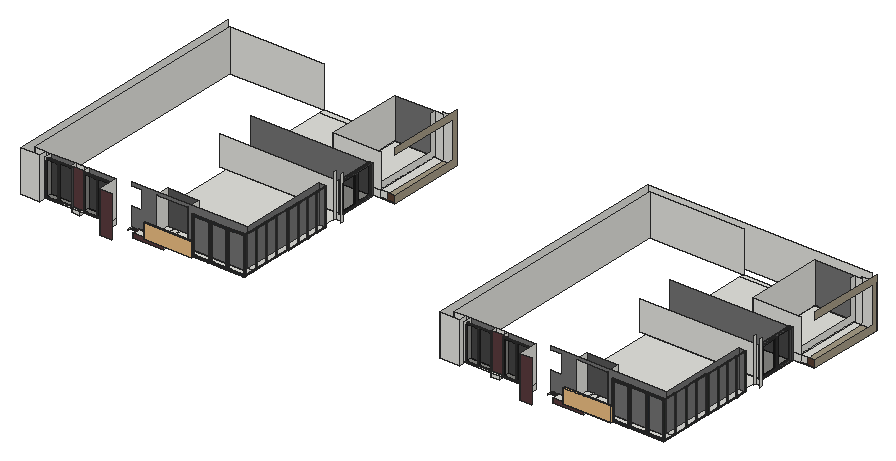
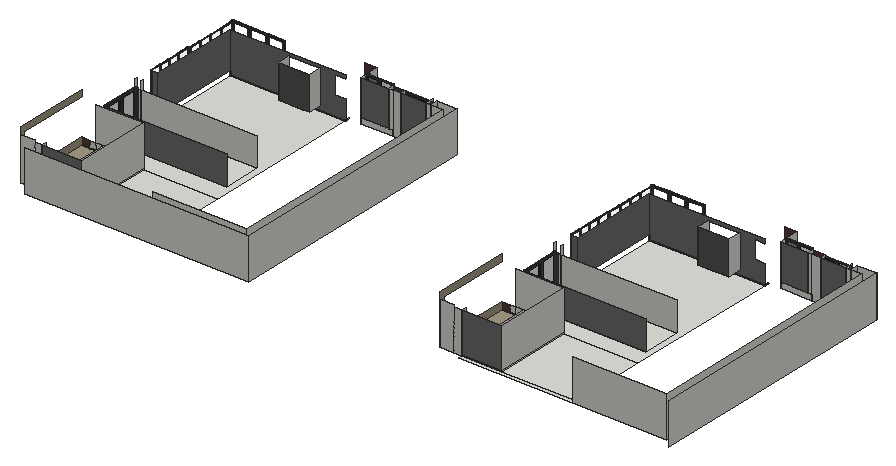
# SketchUp Ruby script. Lengths in inches.
U = 1.inch
M = Sketchup.active_model
def pt(a) = Geom::Point3d.new(a.map { |v| v * U })
def face(e, loops, mat)
  f = e.add_face(loops[0].map { |a| pt(a) })
  loops[1..].each { |l| e.add_face(l.map { |a| pt(a) }).erase! }
  f.material = f.back_material = mat if mat
  f
end
# faces: each face lists its corners as indices into pts; further lists are holes
def faces(e, pts, list, mat = nil) = list.each { |f| face(e, (f[0].is_a?(Array) ? f : [f]).map { |l| l.map { |i| pts[i] } }, mat) }
# xy, xz, yz: faces in a plane at the given z, y or x. An outline is a flat list of corners, or four numbers for a rectangle; further outlines are holes
def ring(l) = l.size == 4 ? [[l[0], l[1]], [l[2], l[1]], [l[2], l[3]], [l[0], l[3]]] : l.each_slice(2).to_a
def flat(e, list, mat, &to3) = list.each { |f| face(e, (f[0].is_a?(Array) ? f : [f]).map { |l| ring(l).map { |u, v| to3.(u, v) } }, mat) }
def xy(e, z, list, mat = nil) = flat(e, list, mat) { |x, y| [x, y, z] }
def xz(e, y, list, mat = nil) = flat(e, list, mat) { |x, z| [x, y, z] }
def yz(e, x, list, mat = nil) = flat(e, list, mat) { |y, z| [x, y, z] }
def lines(e, pts, list) = list.each { |a, b| e.add_line(pt(pts[a]), pt(pts[b])) }
# prism: a flat outline (further loops are holes) pulled along v
def prism(e, loops, v, mat = nil)
  f = face(e, loops, mat); d = Geom::Vector3d.new(v.map { |x| x * U })
  f.pushpull(f.normal.samedirection?(d) ? d.length : -d.length)
end
def box(e, o, s, mat = nil) = prism(e, [[o, [o[0] + s[0], o[1], o[2]], [o[0] + s[0], o[1] + s[1], o[2]], [o[0], o[1] + s[1], o[2]]]], [0, 0, s[2]], mat)
def at(x, y, z, deg = 0) = Geom::Transformation.translation(pt([x, y, z])) * Geom::Transformation.rotation(ORIGIN, Z_AXIS, deg.degrees)
def axes(o, x, y, z) = Geom::Transformation.new([*x, 0, *y, 0, *z, 0, *pt(o).to_a, 1])
def part(name) = M.definitions.add(name)
# library, detail: a bought-in or finely detailed component or shape, given as its bounding box
def library(name, o, s) = part(name).tap { |d| box(d.entities, o, s) }
def detail(e, o, s) = box(e.add_group.entities, o, s)
def put(e, d, t, mat = nil) = e.add_instance(d, t).tap { |i| i.material = mat if mat }
def group(e, t, mat = nil) = e.add_group.tap { |g| g.transformation = t; g.material = mat if mat }.entities
root = M.entities
M.materials.add("Glass_Tinted_Gray").color = [0, 0, 0]
M.materials["Glass_Tinted_Gray"].alpha = 0.125
M.materials.add("Glazing").color = [128, 128, 128]
M.materials["Glazing"].alpha = 0.05
M.materials.add("Powdercoating").color = [41, 44, 40]
M.materials.add("Wine2").color = [0, 0, 0]
M.materials["Wine2"].alpha = 0
M.materials.add("[0130_Gainsboro]").color = [39, 45, 50]
M.materials.add("[0135_DarkGray]").color = [81, 81, 81]
M.materials.add("[Color M05]").color = [114, 114, 114]
M.materials.add("[Color M06]").color = [86, 86, 86]
M.materials.add("[Concrete Tile]").color = [165, 155, 133]
M.materials.add("[Granite Brown]").color = [89, 59, 61]
M.materials.add("[Granite Brown]1").color = [89, 63, 50]
M.materials.add("[Mirror 02]").color = [229, 229, 229]
M.materials.add("[Terrazzo Light Blue]").color = [196, 214, 227]
c1 = library("Glass Railing",[0,0,0],[139.5,4.76,42])
c2 = part("Framed glazing panel")
xy(c2.entities,0,[[0,-0.98,43.07,0],[0,0,43.07,1.4]],"[0130_Gainsboro]")
xy(c2.entities,0.3,[[0.3,-1.43,42.77,-0.98]],"[0130_Gainsboro]")
xy(c2.entities,2.95,[[2.95,-1.43,40.12,-0.63],[2.95,-0.63,40.12,0],[2.95,0,40.12,0.64],[2.95,0.64,40.12,1.4]],"[0130_Gainsboro]")
xy(c2.entities,3.54,[[3.54,-0.63,39.53,0],[3.54,0,39.53,0.64]],"[0130_Gainsboro]")
xy(c2.entities,111.8125,[[3.54,-0.63,39.53,0],[3.54,0,39.53,0.64]],"[0130_Gainsboro]")
xy(c2.entities,112.4,[[2.95,-1.43,40.12,-0.63],[2.95,-0.63,40.12,0],[2.95,0,40.12,0.64],[2.95,0.64,40.12,1.4]],"[0130_Gainsboro]")
xy(c2.entities,115.05,[[0.3,-1.43,42.77,-0.98]],"[0130_Gainsboro]")
xy(c2.entities,115.35,[[0,-0.98,43.07,0],[0,0,43.07,1.4]],"[0130_Gainsboro]")
xz(c2.entities,-1.43,[[[0.3,0.3,42.77,115.05],[2.95,2.95,40.12,112.4]]],"[0130_Gainsboro]")
xz(c2.entities,-0.98,[[[0,0,43.07,115.35],[0.3,0.3,42.77,115.05]]],"[0130_Gainsboro]")
xz(c2.entities,-0.63,[[[2.95,2.95,40.12,112.4],[3.54,3.54,39.53,111.8125]]],"[0130_Gainsboro]")
xz(c2.entities,0,[[3.54,3.54,39.53,111.8125]],"Wine2")
xz(c2.entities,0,[[[0,0,43.07,115.35],[2.95,2.95,40.12,112.4]],[[2.95,2.95,40.12,112.4],[3.54,3.54,39.53,111.8125]]],"[0130_Gainsboro]")
xz(c2.entities,0.64,[[[2.95,2.95,40.12,112.4],[3.54,3.54,39.53,111.8125]]],"[0130_Gainsboro]")
xz(c2.entities,1.4,[[[0,0,43.07,115.35],[2.95,2.95,40.12,112.4]]],"[0130_Gainsboro]")
yz(c2.entities,0,[[-0.98,0,0,115.35],[0,0,1.4,115.35]],"[0130_Gainsboro]")
yz(c2.entities,0.3,[[-1.43,0.3,-0.98,115.05]],"[0130_Gainsboro]")
yz(c2.entities,2.95,[[-1.43,2.95,-0.63,112.4],[-0.63,2.95,0,112.4],[0,2.95,0.64,112.4],[0.64,2.95,1.4,112.4]],"[0130_Gainsboro]")
yz(c2.entities,3.54,[[-0.63,3.54,0,111.8125],[0,3.54,0.64,111.8125]],"[0130_Gainsboro]")
yz(c2.entities,39.53,[[-0.63,3.54,0,111.8125],[0,3.54,0.64,111.8125]],"[0130_Gainsboro]")
yz(c2.entities,40.12,[[-1.43,2.95,-0.63,112.4],[-0.63,2.95,0,112.4],[0,2.95,0.64,112.4],[0.64,2.95,1.4,112.4]],"[0130_Gainsboro]")
yz(c2.entities,42.77,[[-1.43,0.3,-0.98,115.05]],"[0130_Gainsboro]")
yz(c2.entities,43.07,[[-0.98,0,0,115.35],[0,0,1.4,115.35]],"[0130_Gainsboro]")
c3 = part("Glazed panel assembly")
put(c3.entities,c2,axes([90.57,1.43,0],[1.05148,0,0],[0,1,0],[0,0,1]))
put(c3.entities,c2,axes([0,1.43,0],[1.05148,0,0],[0,1,0],[0,0,1]))
put(c3.entities,c2,axes([45.29,1.43,0],[1.05148,0,0],[0,1,0],[0,0,1]))
c4 = part("PENTEK_RP Fineline 50S_Sliding_DoorCase_E1")
box(c4.entities,[0,0,0],[1.51,3.66,99.27],"[0135_DarkGray]")
c5 = part("PENTEK_RP Fineline 50S_SlidingDooe_Case_E2")
box(c5.entities,[0,0,0],[96.25,3.66,1.51],"[0135_DarkGray]")
c6 = part("pentek_RP Fineline 50S_SlidingDoor_Case")
put(c6.entities,c4,at(97.76,0,0))
put(c6.entities,c5,at(1.51,0,0))
put(c6.entities,c4,at(0,0,0))
put(c6.entities,c5,at(1.51,0,97.76))
c7 = part("PENTEK_RP Fineline 50S_SlidingDoor_GlazingBead_2")
box(c7.entities,[0,0,0],[0.56,0.59,94.39],"[0135_DarkGray]")
c8 = part("PENTEK_RP Fineline 50S_SlidingDoor_Glass")
box(c8.entities,[0,0,0],[46.58,0.16,94.39],"Glass_Tinted_Gray")
c9 = part("PENTEK_RP Fineline 50S_SlidingDoor_GlazingBead")
box(c9.entities,[0,0,0],[45.47,0.59,0.56],"[0135_DarkGray]")
c10 = part("PENTEK_RP Fineline 50S_SlidingDoor_Leaf_E1")
xy(c10.entities,0,[[0,0,0.93,1.97],[0.93,1.57,1.49,1.97]],"[0135_DarkGray]")
xy(c10.entities,96.25,[[0,0,0.93,0,0.93,1.57,1.49,1.57,1.49,1.97,0,1.97]],"[0135_DarkGray]")
xz(c10.entities,0,[[0,0,0.93,96.25]],"[0135_DarkGray]")
xz(c10.entities,1.57,[[0.93,0,1.49,95.32],[0.93,95.32,1.49,96.25]],"[0135_DarkGray]")
xz(c10.entities,1.97,[[0,0,1.49,96.25]],"[0135_DarkGray]")
yz(c10.entities,0,[[0,0,1.97,96.25]],"[0135_DarkGray]")
yz(c10.entities,0.93,[[0,0,1.57,0.93],[0,0.93,1.57,95.32],[0,95.32,1.57,96.25]],"[0135_DarkGray]")
yz(c10.entities,1.49,[[1.57,0,1.97,95.32],[1.57,95.32,1.97,96.25]],"[0135_DarkGray]")
c11 = part("PENTEK_RP Fineline 50S_SlidingDoor_Leaf_E2")
xy(c11.entities,0,[[0,0,0,1.57,0.56,1.57,0.56,1.97,46.02,1.97,46.02,1.57,46.58,1.57,46.58,0]],"[0135_DarkGray]")
xy(c11.entities,0.93,[[0,0,46.58,1.57]],"[0135_DarkGray]")
xy(c11.entities,1.49,[[0.56,1.57,46.02,1.97]],"[0135_DarkGray]")
xz(c11.entities,0,[[0,0,46.58,0.93]],"[0135_DarkGray]")
xz(c11.entities,1.57,[[0,0,0.56,0.93],[46.02,0,46.58,0.93],[0.56,0.93,46.02,1.49]],"[0135_DarkGray]")
xz(c11.entities,1.97,[[0.56,0,46.02,1.49]],"[0135_DarkGray]")
yz(c11.entities,0,[[0,0,1.57,0.93]],"[0135_DarkGray]")
yz(c11.entities,0.56,[[1.57,0,1.97,0.93],[1.57,0.93,1.97,1.49]],"[0135_DarkGray]")
yz(c11.entities,46.02,[[1.57,0,1.97,0.93],[1.57,0.93,1.97,1.49]],"[0135_DarkGray]")
yz(c11.entities,46.58,[[0,0,1.57,0.93]],"[0135_DarkGray]")
c12 = part("PENTEK_RP Fineline S_SlidingDoor_Leaf1")
put(c12.entities,c7,at(0.93,0,0.93))
put(c12.entities,c7,at(46.96,0,0.93))
put(c12.entities,c8,at(1.49,1.42,0.93))
put(c12.entities,c9,at(1.49,0,0.93))
put(c12.entities,c8,at(1.49,0.59,0.93),"[Terrazzo Light Blue]")
put(c12.entities,c10,at(0,0,0))
put(c12.entities,c10,axes([48.44,0,0],[-1,0,0],[0,1,0],[0,0,1]))
put(c12.entities,c11,axes([0.93,0,96.25],[1,0,0],[0,1,0],[0,0,-1]))
put(c12.entities,c11,at(0.93,0,0))
put(c12.entities,c9,at(1.49,0,94.77))
c13 = part("PENTEK_RP Fineline 50S_SlidingDoor_Leaf2")
put(c13.entities,c8,at(1.49,1.42,0.93))
put(c13.entities,c9,at(1.49,0,94.77))
put(c13.entities,c7,at(46.96,0,0.93))
put(c13.entities,c8,at(1.49,0.59,0.93),"[Mirror 02]")
put(c13.entities,c7,at(0.93,0,0.93))
put(c13.entities,c10,at(0,0,0))
put(c13.entities,c10,axes([48.44,0,0],[-1,0,0],[0,1,0],[0,0,1]))
put(c13.entities,c9,at(1.49,0,0.93))
put(c13.entities,c11,axes([0.93,0,96.25],[1,0,0],[0,1,0],[0,0,-1]))
put(c13.entities,c11,at(0.93,0,0))
c14 = part("PENTEK - Slimmest Steel Sliding Door / Window\#1")
put(c14.entities,c6,at(0,-1.88,-0.09))
put(c14.entities,c12,at(1.51,-2.27,1.42))
put(c14.entities,c13,at(49.32,-0.3,1.42))
c15 = part("Group\#15")
xy(c15.entities,0,[[0,-55.94,0.71,45.94]])
xy(c15.entities,0.2,[[0,-55.94,0.47,45.94],[0.47,45.94,0.71,46.42]])
xy(c15.entities,2.36,[[0.47,-55.94,0.71,46.42]])
xz(c15.entities,-55.94,[[0,0,0.71,0,0.71,2.36,0.47,2.36,0.47,0.2,0,0.2]])
xz(c15.entities,45.94,[[0,0,0.71,0.2]])
xz(c15.entities,46.42,[[0.47,0.2,0.71,2.36]])
yz(c15.entities,0,[[-55.94,0,45.94,0.2]])
yz(c15.entities,0.47,[[-55.94,0.2,46.42,2.36]])
yz(c15.entities,0.71,[[-55.94,0,45.94,0,45.94,0.2,46.42,0.2,46.42,2.36,-55.94,2.36]])
c16 = part("Group\#7")
xy(c16.entities,0,[[0,-59.09,0.71,45.94]])
xy(c16.entities,0.2,[[0,-59.09,0.47,45.94],[0.47,45.94,0.71,46.42]])
xy(c16.entities,2.36,[[0.47,-59.09,0.71,46.42]])
xz(c16.entities,-59.09,[[0,0,0.71,0,0.71,2.36,0.47,2.36,0.47,0.2,0,0.2]])
xz(c16.entities,45.94,[[0,0,0.71,0.2]])
xz(c16.entities,46.42,[[0.47,0.2,0.71,2.36]])
yz(c16.entities,0,[[-59.09,0,45.94,0.2]])
yz(c16.entities,0.47,[[-59.09,0.2,46.42,2.36]])
yz(c16.entities,0.71,[[-59.09,0,45.94,0,45.94,0.2,46.42,0.2,46.42,2.36,-59.09,2.36]])
c17 = part("Group\#16")
prism(c17.entities,[[[0.47,-56.18,0.2],[0,-56.18,0.2],[0,-56.18,0],[0.71,-56.18,0],[0.71,-56.18,2.36],[0.47,-56.18,2.36]]],[0,28.68,0])
c18 = part("Group\#10")
box(c18.entities,[-0.73,0,0],[27.99,0.55,102.05])
c19 = part("Group\#18")
xy(c19.entities,0,[[0.47,-56.18,0.47,-55.47,0,-55.47,0,-28.21,1.18,-28.21,1.18,-56.18]])
xy(c19.entities,0.2,[[0.71,-56.18,1.18,-28.21],[0,-55.47,0.47,-28.21],[0.47,-28.21,0.71,-27.74]])
xy(c19.entities,2.36,[[0.47,-56.18,0.71,-27.74]])
xz(c19.entities,-56.18,[[0.47,0,1.18,0,1.18,0.2,0.71,0.2,0.71,2.36,0.47,2.36]])
xz(c19.entities,-55.47,[[0,0,0.47,0.2]])
xz(c19.entities,-28.21,[[0,0,1.18,0.2]])
xz(c19.entities,-27.74,[[0.47,0.2,0.71,2.36]])
yz(c19.entities,0,[[-55.47,0,-28.21,0.2]])
yz(c19.entities,0.47,[[-56.18,0,-55.47,0.2],[-56.18,0.2,-27.74,2.36]])
yz(c19.entities,0.71,[[-56.18,0.2,-27.74,2.36]])
yz(c19.entities,1.18,[[-56.18,0,-28.21,0.2]])
c20 = part("Group\#34")
xy(c20.entities,0,[[-20.45,0,7.76,1.22]])
xy(c20.entities,0.06,[[-20.39,0.06,7.7,1.22]])
xy(c20.entities,0.47,[[-19.98,0,7.28,0.06]])
xy(c20.entities,101.89,[[-19.98,0,7.28,0.06]])
xy(c20.entities,102.3,[[-20.39,0.06,7.7,1.22]])
xy(c20.entities,102.36,[[-20.45,0,7.76,1.22]])
xz(c20.entities,0,[[[-20.45,0,7.76,102.36],[-19.98,0.47,7.28,101.89]]])
xz(c20.entities,0.06,[[[-20.39,0.06,7.7,102.3],[-19.98,0.47,7.28,101.89]]])
xz(c20.entities,1.22,[[[-20.45,0,7.76,102.36],[-20.39,0.06,7.7,102.3]]])
yz(c20.entities,-20.45,[[0,0,1.22,102.36]])
yz(c20.entities,-20.39,[[0.06,0.06,1.22,102.3]])
yz(c20.entities,-19.98,[[0,0.47,0.06,101.89]])
yz(c20.entities,7.28,[[0,0.47,0.06,101.89]])
yz(c20.entities,7.7,[[0.06,0.06,1.22,102.3]])
yz(c20.entities,7.76,[[0,0,1.22,102.36]])
c21 = part("Group\#6")
put(c21.entities,c15,axes([27.97,0,7.875],[1,0,0],[0,0,-1],[0,1,0]),"Powdercoating")
put(c21.entities,c16,axes([0.71,0,6.8],[-1,0,0],[0,0,-0.97687],[0,1,0]),"Powdercoating")
put(c21.entities,c17,axes([-27.5,0,-38.07],[0,0,-1],[-1,0,0],[0,1,0]),"Powdercoating")
put(c21.entities,c18,at(1.12,0.35,-38.39),"Glazing")
put(c21.entities,c19,axes([-27.5,0,63.35],[0,0,1],[-1,0,0],[0,1,0]),"Powdercoating")
put(c21.entities,c20,at(20.6875,1.0625,-38.54),"Powdercoating")
c22 = part("Sliding door assembly")
put(c22.entities,c21,at(-1.18,4.5,38.86))
g1 = group(c22.entities,at(84.74,4.5,38.86))
put(g1,c15,axes([-27.97,0,7.875],[-1,0,0],[0,0,-1],[0,1,0]),"Powdercoating")
put(g1,c16,axes([-0.71,0,6.8],[1,0,0],[0,0,-0.97687],[0,1,0]),"Powdercoating")
put(g1,c17,axes([27.5,0,-38.07],[0,0,-1],[1,0,0],[0,1,0]),"Powdercoating")
put(g1,c18,axes([-1.12,0.35,-38.39],[-1,0,0],[0,1,0],[0,0,1]),"Glazing")
put(g1,c19,axes([27.5,0,63.35],[0,0,1],[1,0,0],[0,1,0]),"Powdercoating")
put(g1,c20,axes([-20.6875,1.0625,-38.54],[-1,0,0],[0,1,0],[0,0,1]),"Powdercoating")
g2 = group(c22.entities,at(56.0625,4.5,38.86))
put(g2,c15,axes([-27.97,0,7.875],[-1,0,0],[0,0,-1],[0,1,0]),"Powdercoating")
put(g2,c17,axes([27.5,0,-38.07],[0,0,-1],[1,0,0],[0,1,0]),"Powdercoating")
put(g2,c18,axes([-1.12,0.35,-38.39],[-1,0,0],[0,1,0],[0,0,1]),"Glazing")
put(g2,c19,axes([27.5,0,63.35],[0,0,1],[1,0,0],[0,1,0]),"Powdercoating")
put(g2,c20,axes([-20.6875,1.0625,-38.54],[-1,0,0],[0,1,0],[0,0,1]),"Powdercoating")
g3 = group(g2,at(-0.71,0,6.8),"Powdercoating")
xy(g3,-45.34,[[0.47,0.2,0.71,2.36]])
xy(g3,-44.88,[[0,0,0.71,0.2]])
xy(g3,57.73,[[0,0,0.71,0,0.71,2.36,0.47,2.36,0.47,0.2,0,0.2]])
xz(g3,0,[[0,-44.88,0.71,57.73]])
xz(g3,0.2,[[0.47,-45.34,0.71,-44.88],[0,-44.88,0.47,57.73]])
xz(g3,2.36,[[0.47,-45.34,0.71,57.73]])
yz(g3,0,[[0,-44.88,0.2,57.73]])
yz(g3,0.47,[[0.2,-45.34,2.36,57.73]])
yz(g3,0.71,[[0.2,-45.34,2.36,-45.34,2.36,57.73,0,57.73,0,-44.88,0.2,-44.88]])
put(c22.entities,c21,axes([-33.94,4.5,38.86],[1.14218,0,0],[0,1,0],[0,0,1]))
c23 = part("sliding door")
put(c23.entities,c22,at(0,-4.5,-0.08))
xy(root,1518,[[589.7,1799.9375,679.51,1822.9375],[1807.88,1799.9375,1897.7,1822.9375],[557.88,1822.9375,558.625,1835.1875],[679.51,1822.9375,890.875,1829],[1776.07,1822.9375,1776.8125,1835.1875],
  [1897.7,1822.9375,2109.0625,1829],[558.625,1829,679.51,1835.1875],[679.51,1829,890.875,1835.1875],[1776.8125,1829,1897.7,1835.1875],[1897.7,1829,2109.0625,1835.1875],
  [558.625,1835.1875,890.875,2295.875],[1776.8125,1835.1875,2109.0625,2295.875],[558.625,2295.875,774.6875,2518.89],[774.6875,2295.875,890.875,2518.89],[890.875,2295.875,913.875,2518.89],
  [1776.8125,2295.875,1992.875,2518.89],[1992.875,2295.875,2109.0625,2518.89],[2109.0625,2295.875,2132.0625,2518.89],[558.625,2518.89,890.875,2531.375],[1776.8125,2518.89,2109.0625,2531.375]])
xy(root,1518,[[913.875,2295.875,954.6875,2518.89],[2132.0625,2295.875,2172.875,2518.89]],"[Concrete Tile]")
xy(root,1518,[[557.4,1822.9375,557.88,1835.1875],[1775.59,1822.9375,1776.07,1835.1875]],"[Granite Brown]")
xy(root,1519.75,[[774.6875,2295.875,890.875,2518.89],[1992.875,2295.875,2109.0625,2518.89]])
xy(root,1519.8125,[[558.625,1829,890.875,1835.1875],[1776.8125,1829,2109.0625,1835.1875]])
xy(root,1530.6875,[[589.7,1799.9375,679.51,1822.9375],[679.51,1799.9375,913.875,1799.9375,913.875,1835.1875,890.875,1835.1875,890.875,1822.9375,679.51,1822.9375],[1807.88,1799.9375,1897.7,1822.9375],[1897.7,1799.9375,2132.0625,1799.9375,2132.0625,1835.1875,2109.0625,1835.1875,2109.0625,1822.9375,1897.7,1822.9375],[894.3125,1835.1875,913.875,2094.15],
  [2112.5,1835.1875,2132.0625,2094.15]])
xy(root,1531.38,[[652.3,1835.1875,668.6,1873.375],[668.6,1835.1875,670.29,1873.375],[670.29,1835.1875,721.4,1873.375],[1870.49,1835.1875,1886.79,1873.375],[1886.79,1835.1875,1888.48,1873.375],
  [1888.48,1835.1875,1939.59,1873.375]])
xy(root,1531.7,[[631.46,1835.1875,652.3,1873.375],[1849.65,1835.1875,1870.49,1873.375]])
xy(root,1533.4375,[[333.68,1799.9375,523.04,1799.9375,523.04,1822.9375,442.15,1822.9375,442.15,1806.5625,406.21,1806.5625,406.21,1822.9375,333.68,1822.9375],[1551.87,1799.9375,1741.23,1799.9375,1741.23,1822.9375,1660.33,1822.9375,1660.33,1806.5625,1624.4,1806.5625,1624.4,1822.9375,1551.87,1822.9375],[431.33,1806.5625,442.15,1822.9375],[1649.52,1806.5625,1660.33,1822.9375]])
xy(root,1535.36,[[558.625,2156.01,913.875,2266.33],[1776.8125,2156.01,2132.0625,2266.33]])
xz(root,1763.25,[[523.04,1518,557.88,1638],[1741.23,1518,1776.07,1638]],"[Granite Brown]")
xz(root,1799.9375,[[262.875,1518,319.53,1638],[1481.0625,1518,1537.72,1638]])
xz(root,1799.9375,[[589.7,1518,679.51,1530.6875],[1807.88,1518,1897.7,1530.6875]],"[Granite Brown]")
xz(root,1806.5625,[[406.21,1518,406.21,1533.4375,406.29,1533.4375],[406.21,1518,431.33,1518,431.33,1533.4375,406.29,1533.4375],[1624.4,1518,1624.4,1533.4375,1624.48,1533.4375],[1624.4,1518,1649.52,1518,1649.52,1533.4375,1624.48,1533.4375]])
xz(root,1806.5625,[[406.29,1533.4375,442.15,1533.4375,442.15,1638,406.8125,1638],[1624.48,1533.4375,1660.33,1533.4375,1660.33,1638,1625,1638]],"[Granite Brown]")
xz(root,1822.9375,[[285.875,1518,319.53,1638],[319.53,1518,406.21,1518,406.21,1533.4375,333.68,1533.4375,333.68,1638,319.53,1638],[406.21,1518,406.8125,1638,431.33,1638,431.33,1518],[431.33,1518,523.04,1533.4375],[589.7,1518,679.51,1530.6875],
  [679.51,1518,890.875,1530.6875],[1504.0625,1518,1537.72,1638],[1537.72,1518,1624.4,1518,1624.4,1533.4375,1551.87,1533.4375,1551.87,1638,1537.72,1638],[1624.4,1518,1625,1638,1649.52,1638,1649.52,1518],[1649.52,1518,1741.23,1533.4375],
  [1807.88,1518,1897.7,1530.6875],[1897.7,1518,2109.0625,1530.6875],[431.33,1533.4375,442.15,1638],[1649.52,1533.4375,1660.33,1638]])
xz(root,1822.9375,[[406.21,1518,406.8125,1638,333.68,1638,333.68,1533.4375,406.21,1533.4375],[1624.4,1518,1625,1638,1551.87,1638,1551.87,1533.4375,1624.4,1533.4375],[442.15,1533.4375,523.04,1638],[1660.33,1533.4375,1741.23,1638]],"[Color M05]")
xz(root,1829,[[558.625,1518,890.875,1519.8125],[1776.8125,1518,2109.0625,1519.8125]])
xz(root,1835.1875,[[558.625,1518,890.875,1519.8125],[890.875,1518,894.3125,1530.6875],[1776.8125,1518,2109.0625,1519.8125],[2109.0625,1518,2112.5,1530.6875]])
xz(root,1835.1875,[[[557.88,1518,558.625,1518,558.625,1519.8125,890.875,1519.8125,890.875,1530.6875,894.3125,1530.6875,894.3125,1638,557.88,1638,557.88,1627.45,588.66,1627.45,588.66,1575.17,557.88,1575.17],[652.3,1531.38,652.3,1531.7,631.46,1531.7,631.46,1629.51,721.4,1629.51,721.4,1531.38]],[[1776.07,1518,1776.8125,1518,1776.8125,1519.8125,2109.0625,1519.8125,2109.0625,1530.6875,2112.5,1530.6875,2112.5,1638,1776.07,1638,1776.07,1627.45,1806.84,1627.45,1806.84,1575.17,1776.07,1575.17],[1870.49,1531.38,1870.49,1531.7,1849.65,1531.7,1849.65,1629.51,1939.59,1629.51,1939.59,1531.38]]],"[Color M05]")
xz(root,1873.375,[[652.3,1531.38,721.4,1531.38,721.4,1629.51,631.46,1629.51,631.46,1531.7,652.3,1531.7],[1870.49,1531.38,1939.59,1531.38,1939.59,1629.51,1849.65,1629.51,1849.65,1531.7,1870.49,1531.7]],"[Color M06]")
xz(root,2094.15,[[894.3125,1530.6875,913.875,1638],[2112.5,1530.6875,2132.0625,1638]],"[Color M05]")
xz(root,2156.01,[[894.3125,1518,913.875,1535.36],[2112.5,1518,2132.0625,1535.36],[558.625,1535.36,894.3125,1621.04],[894.3125,1535.36,913.875,1621.04],[1776.8125,1535.36,2112.5,1621.04],
  [2112.5,1535.36,2132.0625,1621.04],[2112.5,1535.36,2132.0625,1621.04]])
xz(root,2266.33,[[558.625,1535.36,913.875,1621.04],[1776.8125,1535.36,2132.0625,1621.04]],"[Color M05]")
xz(root,2295.875,[[774.6875,1518,890.875,1519.75],[890.875,1518,913.875,1538.8125],[913.875,1518,930.75,1519.75],[930.75,1518,954.6875,1519.75],[1992.875,1518,2109.0625,1519.75],
  [2109.0625,1518,2132.0625,1538.8125],[2132.0625,1518,2148.9375,1519.75],[2148.9375,1518,2172.875,1519.75],[774.6875,1519.75,774.6875,1638,913.875,1638,913.875,1538.8125,890.875,1538.8125,890.875,1519.75],[913.875,1519.75,930.75,1538.8125],
  [1992.875,1519.75,1992.875,1638,2132.0625,1638,2132.0625,1538.8125,2109.0625,1538.8125,2109.0625,1519.75],[2132.0625,1519.75,2148.9375,1538.8125]])
xz(root,2295.875,[[930.75,1519.75,954.6875,1538.8125],[2148.9375,1519.75,2172.875,1538.8125]],"[Granite Brown]1")
xz(root,2518.89,[[774.6875,1518,890.875,1519.75],[890.875,1518,913.875,1638],[913.875,1518,954.6875,1643.375],[1992.875,1518,2109.0625,1519.75],[2109.0625,1518,2132.0625,1638],
  [2132.0625,1518,2172.875,1643.375]])
xz(root,2518.89,[[774.6875,1519.75,890.875,1638],[1992.875,1519.75,2109.0625,1638]],"[Color M05]")
xz(root,2531.375,[[285.875,1518,558.625,1638],[1504.0625,1518,1776.8125,1638]])
xz(root,2554.375,[[1481.0625,1518,2132.0625,1638]])
yz(root,262.875,[[1799.9375,1518,2554.375,1638]])
yz(root,285.875,[[1822.9375,1518,2531.375,1638]])
yz(root,319.53,[[1799.9375,1518,1822.9375,1638]])
yz(root,333.68,[[1799.9375,1533.4375,1822.9375,1638]])
yz(root,406.21,[[1806.5625,1518,1822.9375,1533.4375]])
yz(root,431.33,[[1806.5625,1518,1822.9375,1533.4375]])
yz(root,442.15,[[1806.5625,1533.4375,1822.9375,1638]])
yz(root,523.04,[[1763.25,1518,1799.9375,1533.4375],[1799.9375,1518,1822.9375,1533.4375],[1763.25,1533.4375,1822.9375,1638]])
yz(root,558.625,[[1822.9375,1518,1829,1519.8125],[1829,1518,1835.1875,1519.8125]])
yz(root,589.7,[[1799.9375,1518,1822.9375,1530.6875]],"[Granite Brown]")
yz(root,631.46,[[1835.1875,1531.7,1873.375,1629.51]])
yz(root,652.3,[[1835.1875,1531.38,1873.375,1531.7]])
yz(root,679.51,[[1799.9375,1518,1822.9375,1530.6875]])
yz(root,721.4,[[1835.1875,1531.38,1873.375,1629.51]])
yz(root,774.6875,[[2295.875,1518,2518.89,1519.75],[2295.875,1519.75,2518.89,1638]])
yz(root,890.875,[[1822.9375,1518,1829,1530.6875],[1829,1518,1835.1875,1519.8125],[2295.875,1518,2518.89,1519.75],[2295.875,1519.75,2295.875,1538.8125,2505.21,1538.8125,2505.21,1638,2518.89,1638,2518.89,1519.75],[1829,1519.8125,1835.1875,1530.6875]])
yz(root,894.3125,[[2148.83,1518,2156.01,1644]])
yz(root,894.3125,[[1835.1875,1530.6875,2094.15,1638]],"[Color M05]")
yz(root,913.875,[[2148.83,1518,2156.01,1644]])
yz(root,954.6875,[[2295.875,1518,2518.89,1518,2518.89,1663.0625,2295.875,1663.0625,2295.875,1643.375,2505.21,1643.375,2505.21,1538.8125,2295.875,1538.8125]],"[Concrete Tile]")
yz(root,1481.0625,[[1799.9375,1518,2554.375,1638]])
yz(root,1504.0625,[[1822.9375,1518,2531.375,1638]])
yz(root,1537.72,[[1799.9375,1518,1822.9375,1638]])
yz(root,1551.87,[[1799.9375,1533.4375,1822.9375,1638]])
yz(root,1624.4,[[1806.5625,1518,1822.9375,1533.4375]])
yz(root,1649.52,[[1806.5625,1518,1822.9375,1533.4375]])
yz(root,1660.33,[[1806.5625,1533.4375,1822.9375,1638]])
yz(root,1741.23,[[1763.25,1518,1799.9375,1533.4375],[1799.9375,1518,1822.9375,1533.4375],[1763.25,1533.4375,1822.9375,1638]])
yz(root,1776.8125,[[1822.9375,1518,1829,1519.8125],[1829,1518,1835.1875,1519.8125]])
yz(root,1807.88,[[1799.9375,1518,1822.9375,1530.6875]],"[Granite Brown]")
yz(root,1849.65,[[1835.1875,1531.7,1873.375,1629.51]])
yz(root,1870.49,[[1835.1875,1531.38,1873.375,1531.7]])
yz(root,1897.7,[[1799.9375,1518,1822.9375,1530.6875]])
yz(root,1939.59,[[1835.1875,1531.38,1873.375,1629.51]])
yz(root,1992.875,[[2295.875,1518,2518.89,1519.75],[2295.875,1519.75,2518.89,1638]])
yz(root,2109.0625,[[1822.9375,1518,1829,1530.6875],[1829,1518,1835.1875,1519.8125],[2295.875,1518,2518.89,1519.75],[2295.875,1519.75,2295.875,1538.8125,2505.21,1538.8125,2505.21,1638,2518.89,1638,2518.89,1519.75],[1829,1519.8125,1835.1875,1530.6875]])
yz(root,2112.5,[[2148.83,1518,2156.01,1644]])
yz(root,2112.5,[[1835.1875,1530.6875,2094.15,1638]],"[Color M05]")
yz(root,2132.0625,[[2148.83,1518,2156.01,1644]])
yz(root,2172.875,[[2295.875,1518,2518.89,1518,2518.89,1663.0625,2295.875,1663.0625,2295.875,1643.375,2505.21,1643.375,2505.21,1538.8125,2295.875,1538.8125]],"[Concrete Tile]")
p = [[406.21,1822.9375,1518],[406.21,1806.5625,1518],[406.29,1806.5625,1533.4375],[406.8125,1806.5625,1638],[406.8125,1822.9375,1638],[1624.4,1822.9375,1518],
  [1624.4,1806.5625,1518],[1624.48,1806.5625,1533.4375],[1625,1806.5625,1638],[1625,1822.9375,1638]]
faces(root,p,[[0,1,2,3,4],[5,6,7,8,9]])
put(root,c1,at(1840.53,1798.18,1527.4))
put(root,c1,at(622.34,1798.18,1527.4))
put(root,c3,axes([1979.67,1799.9375,1530.6875],[1.12166,0,0],[0,1,0],[0,0,0.95]))
put(root,c3,axes([761.48,1799.9375,1530.6875],[1.12166,0,0],[0,1,0],[0,0,0.95]))
put(root,c14,axes([1664.65,1801.81,1533.53],[0.7714,0,0],[0,1,0],[0,0,1.054]))
put(root,c14,axes([446.46,1801.81,1533.53],[0.7714,0,0],[0,1,0],[0,0,1.054]))
put(root,c14,axes([1550.21,1806.86,1530.375],[0.7714,0,0],[0,1,0],[0,0,1.054]))
put(root,c14,axes([332.02,1806.86,1530.375],[0.7714,0,0],[0,1,0],[0,0,1.054]))
put(root,c23,axes([2132.0625,1844.58,1530.6875],[0,1.302,0],[-1,0,0],[0,0,1.03877]))
put(root,c23,axes([913.875,1844.58,1530.6875],[0,1.302,0],[-1,0,0],[0,0,1.03877]))
put(root,c23,axes([2134.42,1995.73,1531.32],[0,1.13453,0],[-1,0,0],[0,0,1.03262]))
put(root,c23,axes([916.24,1995.73,1531.32],[0,1.13453,0],[-1,0,0],[0,0,1.03262]))
put(root,c14,axes([2126.35,2154.96,1535.4375],[0,1.12181,0],[-2.51374,0,0],[0,0,0.87918]))
put(root,c14,axes([908.17,2154.96,1535.4375],[0,1.12181,0],[-2.51374,0,0],[0,0,0.87918]))
